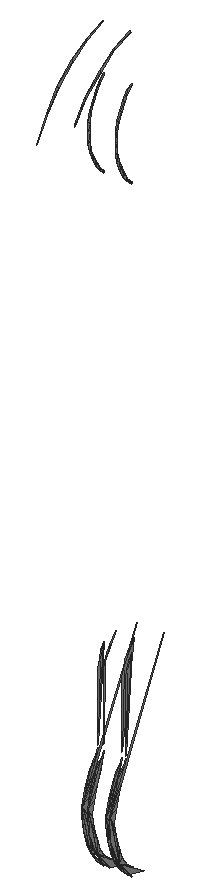
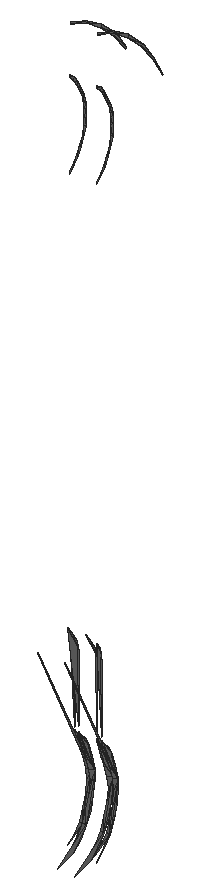
# SketchUp Ruby script. Lengths in inches.
U = 1.inch
M = Sketchup.active_model
def pt(a) = Geom::Point3d.new(a.map { |v| v * U })
def face(e, loops, mat)
  f = e.add_face(loops[0].map { |a| pt(a) })
  loops[1..].each { |l| e.add_face(l.map { |a| pt(a) }).erase! }
  f.material = f.back_material = mat if mat
  f
end
# faces: each face lists its corners as indices into pts; further lists are holes
def faces(e, pts, list, mat = nil) = list.each { |f| face(e, (f[0].is_a?(Array) ? f : [f]).map { |l| l.map { |i| pts[i] } }, mat) }
# xy, xz, yz: faces in a plane at the given z, y or x. An outline is a flat list of corners, or four numbers for a rectangle; further outlines are holes
def ring(l) = l.size == 4 ? [[l[0], l[1]], [l[2], l[1]], [l[2], l[3]], [l[0], l[3]]] : l.each_slice(2).to_a
def flat(e, list, mat, &to3) = list.each { |f| face(e, (f[0].is_a?(Array) ? f : [f]).map { |l| ring(l).map { |u, v| to3.(u, v) } }, mat) }
def xy(e, z, list, mat = nil) = flat(e, list, mat) { |x, y| [x, y, z] }
def xz(e, y, list, mat = nil) = flat(e, list, mat) { |x, z| [x, y, z] }
def yz(e, x, list, mat = nil) = flat(e, list, mat) { |y, z| [x, y, z] }
def lines(e, pts, list) = list.each { |a, b| e.add_line(pt(pts[a]), pt(pts[b])) }
# prism: a flat outline (further loops are holes) pulled along v
def prism(e, loops, v, mat = nil)
  f = face(e, loops, mat); d = Geom::Vector3d.new(v.map { |x| x * U })
  f.pushpull(f.normal.samedirection?(d) ? d.length : -d.length)
end
def box(e, o, s, mat = nil) = prism(e, [[o, [o[0] + s[0], o[1], o[2]], [o[0] + s[0], o[1] + s[1], o[2]], [o[0], o[1] + s[1], o[2]]]], [0, 0, s[2]], mat)
def at(x, y, z, deg = 0) = Geom::Transformation.translation(pt([x, y, z])) * Geom::Transformation.rotation(ORIGIN, Z_AXIS, deg.degrees)
def axes(o, x, y, z) = Geom::Transformation.new([*x, 0, *y, 0, *z, 0, *pt(o).to_a, 1])
def part(name) = M.definitions.add(name)
# library, detail: a bought-in or finely detailed component or shape, given as its bounding box
def library(name, o, s) = part(name).tap { |d| box(d.entities, o, s) }
def detail(e, o, s) = box(e.add_group.entities, o, s)
def put(e, d, t, mat = nil) = e.add_instance(d, t).tap { |i| i.material = mat if mat }
def group(e, t, mat = nil) = e.add_group.tap { |g| g.transformation = t; g.material = mat if mat }.entities
root = M.entities
M.materials.add("Material \#1").color = [140, 140, 140]
yz(root,263.95,[[328.065,58.084,328.018,58.124,327.978,58.176],[328.078,58.12,327.978,58.176,328.037,58.155],[328.037,58.155,327.978,58.176,328.002,58.201],[327.978,58.176,327.924,58.431,327.958,58.319],[327.978,58.176,327.929,58.31,327.924,58.431],
  [327.978,58.176,327.948,58.239,327.929,58.31],[327.978,58.176,327.958,58.319,327.975,58.256],[327.978,58.176,327.975,58.256,328.002,58.201],[327.929,58.31,327.922,58.387,327.924,58.431],[327.958,58.319,327.924,58.431,327.952,58.387],
  [327.952,58.387,327.924,58.431,327.958,58.455],[327.924,58.431,327.931,58.474,327.941,58.515],[327.924,58.431,327.941,58.515,327.973,58.588],[327.924,58.431,327.973,58.588,328.022,58.654],[327.924,58.431,327.975,58.517,327.958,58.455],
  [327.924,58.431,328.002,58.572,327.975,58.517],[327.924,58.431,328.022,58.654,328.026,58.66],[327.924,58.431,328.026,58.66,328.029,58.667],[327.924,58.431,328.288,59.173,328.002,58.572],[327.941,58.515,327.955,58.553,327.973,58.588],
  [327.973,58.588,327.994,58.62,328.017,58.648],[327.973,58.588,328.017,58.648,328.022,58.654],[328.034,58.6875,328.035,58.695,328.066,59.173],[328.035,58.695,328.035,59.055,328.038,59.098],[328.035,58.695,328.038,59.098,328.066,59.173],
  [328.038,59.098,328.049,59.138,328.066,59.173]],"Material \#1")
yz(root,263.952,[[328.067,61.457,328.037,61.485,328.044,61.497],[328.067,61.457,328.044,61.497,328.073,61.47],[328.037,61.485,328.011,61.52,328.019,61.53],[328.037,61.485,328.019,61.53,328.044,61.497],[328.011,61.52,327.989,61.56,327.999,61.568],
  [328.011,61.52,327.999,61.568,328.019,61.53],[327.989,61.56,327.973,61.605,327.984,61.61],[327.989,61.56,327.984,61.61,327.999,61.568],[327.973,61.605,327.963,61.654,327.974,61.657],[327.973,61.605,327.974,61.657,327.984,61.61],
  [327.963,61.654,327.959,61.71,327.971,61.71],[327.963,61.654,327.971,61.71,327.974,61.657],[327.959,61.71,327.963,61.757,327.974,61.754],[327.959,61.71,327.974,61.754,327.971,61.71],[327.974,61.754,327.963,61.757,327.984,61.8],
  [327.963,61.757,327.973,61.806,327.984,61.8],[327.984,61.8,327.973,61.806,327.999,61.843],[327.614,61.803,327.676,61.917,327.684,61.907],[327.973,61.806,327.989,61.851,327.999,61.843],[327.999,61.843,327.989,61.851,328.019,61.881],
  [327.989,61.851,328.011,61.891,328.019,61.881],[328.019,61.881,328.011,61.891,328.044,61.914],[328.011,61.891,328.037,61.925,328.044,61.914],[327.684,61.907,327.676,61.917,327.762,62.01],[328.044,61.914,328.037,61.925,328.073,61.941],
  [327.676,61.917,327.755,62.021,327.762,62.01],[328.037,61.925,328.067,61.954,328.073,61.941],[327.762,62.01,327.755,62.021,327.852,62.094],[327.755,62.021,327.846,62.107,327.852,62.094],[327.852,62.094,327.846,62.107,327.952,62.157],
  [327.846,62.107,327.948,62.171,327.952,62.157],[327.952,62.157,327.948,62.171,328.061,62.196],[327.948,62.171,328.059,62.211,328.061,62.196]],"Material \#1")
yz(root,263.975,[[328.177,58.05,327.978,58.176,328.065,58.084],[328.065,58.084,327.978,58.176,328.018,58.124],[328.078,58.12,328.037,58.155,327.978,58.176],[328.037,58.155,328.002,58.201,327.978,58.176],[327.978,58.176,327.924,58.431,327.929,58.31],
  [327.978,58.176,327.975,58.256,327.924,58.431],[327.978,58.176,327.929,58.31,327.948,58.239],[327.978,58.176,328.002,58.201,327.975,58.256],[327.975,58.256,327.958,58.319,327.924,58.431],[327.929,58.31,327.924,58.431,327.922,58.387],
  [327.958,58.319,327.952,58.387,327.924,58.431],[327.952,58.387,327.958,58.455,327.924,58.431],[327.924,58.431,327.941,58.515,327.931,58.474],[327.924,58.431,327.958,58.455,327.975,58.517],[327.924,58.431,327.973,58.588,327.941,58.515],
  [327.924,58.431,327.975,58.517,328.029,58.667],[327.924,58.431,328.022,58.654,327.973,58.588],[327.924,58.431,328.026,58.66,328.022,58.654],[327.924,58.431,328.029,58.667,328.026,58.66],[327.941,58.515,327.973,58.588,327.955,58.553],
  [327.975,58.517,328.002,58.572,328.029,58.667],[327.973,58.588,328.017,58.648,327.994,58.62],[327.973,58.588,328.022,58.654,328.017,58.648],[328.035,58.695,328.038,59.098,328.035,59.055],[328.038,59.098,328.066,59.173,328.049,59.138],
  [328.038,59.098,328.115,59.224,328.066,59.173]],"Material \#1")
yz(root,264.078,[[328.177,58.05,328.065,58.084,327.978,58.176],[328.065,58.084,328.018,58.124,327.978,58.176],[328.078,58.12,327.978,58.176,328.037,58.155],[328.037,58.155,327.978,58.176,328.002,58.201],[327.978,58.176,327.924,58.431,327.975,58.256],
  [327.978,58.176,327.929,58.31,327.924,58.431],[327.978,58.176,327.948,58.239,327.929,58.31],[327.978,58.176,327.975,58.256,328.002,58.201],[327.975,58.256,327.924,58.431,327.958,58.319],[327.929,58.31,327.922,58.387,327.924,58.431],
  [327.958,58.319,327.924,58.431,327.952,58.387],[327.952,58.387,327.924,58.431,327.958,58.455],[327.924,58.431,327.931,58.474,327.941,58.515],[327.924,58.431,327.941,58.515,327.973,58.588],[327.924,58.431,327.973,58.588,328.022,58.654],
  [327.924,58.431,327.975,58.517,327.958,58.455],[327.924,58.431,328.022,58.654,328.026,58.66],[327.924,58.431,328.026,58.66,328.029,58.667],[327.924,58.431,328.029,58.667,327.975,58.517],[327.941,58.515,327.955,58.553,327.973,58.588],
  [327.975,58.517,328.029,58.667,328.002,58.572],[327.973,58.588,327.994,58.62,328.017,58.648],[327.973,58.588,328.017,58.648,328.022,58.654],[328.035,58.695,328.035,59.055,328.038,59.098],[328.035,58.695,328.038,59.098,328.115,59.224],
  [328.038,59.098,328.049,59.138,328.066,59.173],[328.038,59.098,328.066,59.173,328.115,59.224],[328.066,59.173,328.088,59.202,328.115,59.224]],"Material \#1")
yz(root,264.101,[[328.067,61.457,328.044,61.497,328.037,61.485],[328.067,61.457,328.073,61.47,328.044,61.497],[328.037,61.485,328.019,61.53,328.011,61.52],[328.037,61.485,328.044,61.497,328.019,61.53],[328.011,61.52,327.999,61.568,327.989,61.56],
  [328.011,61.52,328.019,61.53,327.999,61.568],[327.989,61.56,327.984,61.61,327.973,61.605],[327.989,61.56,327.999,61.568,327.984,61.61],[327.973,61.605,327.974,61.657,327.963,61.654],[327.973,61.605,327.984,61.61,327.974,61.657],
  [327.963,61.654,327.971,61.71,327.959,61.71],[327.963,61.654,327.974,61.657,327.971,61.71],[327.959,61.71,327.971,61.71,327.974,61.754],[327.959,61.71,327.974,61.754,327.963,61.757],[327.974,61.754,327.984,61.8,327.963,61.757],
  [327.963,61.757,327.984,61.8,327.973,61.806],[327.984,61.8,327.999,61.843,327.973,61.806],[327.973,61.806,327.999,61.843,327.989,61.851],[327.999,61.843,328.019,61.881,327.989,61.851],[327.989,61.851,328.019,61.881,328.011,61.891],
  [328.019,61.881,328.044,61.914,328.011,61.891],[328.011,61.891,328.044,61.914,328.037,61.925],[327.684,61.907,327.762,62.01,327.676,61.917],[328.044,61.914,328.073,61.941,328.037,61.925],[327.676,61.917,327.762,62.01,327.755,62.021],
  [328.037,61.925,328.073,61.941,328.067,61.954],[327.762,62.01,327.852,62.094,327.755,62.021],[327.755,62.021,327.852,62.094,327.846,62.107],[327.852,62.094,327.952,62.157,327.846,62.107],[327.846,62.107,327.952,62.157,327.948,62.171],
  [327.952,62.157,328.061,62.196,327.948,62.171],[327.948,62.171,328.061,62.196,328.059,62.211]],"Material \#1")
yz(root,264.103,[[328.065,58.084,327.978,58.176,328.018,58.124],[328.078,58.12,328.037,58.155,327.978,58.176],[328.037,58.155,328.002,58.201,327.978,58.176],[327.978,58.176,327.924,58.431,327.929,58.31],[327.978,58.176,327.958,58.319,327.924,58.431],
  [327.978,58.176,327.929,58.31,327.948,58.239],[327.978,58.176,327.975,58.256,327.958,58.319],[327.978,58.176,328.002,58.201,327.975,58.256],[327.929,58.31,327.924,58.431,327.922,58.387],[327.958,58.319,327.952,58.387,327.924,58.431],
  [327.952,58.387,327.958,58.455,327.924,58.431],[327.924,58.431,327.941,58.515,327.931,58.474],[327.924,58.431,327.958,58.455,327.975,58.517],[327.924,58.431,327.973,58.588,327.941,58.515],[327.924,58.431,327.975,58.517,328.002,58.572],
  [327.924,58.431,328.002,58.572,328.288,59.173],[327.924,58.431,328.022,58.654,327.973,58.588],[327.924,58.431,328.026,58.66,328.022,58.654],[327.924,58.431,328.029,58.667,328.026,58.66],[327.941,58.515,327.973,58.588,327.955,58.553],
  [327.973,58.588,328.017,58.648,327.994,58.62],[327.973,58.588,328.022,58.654,328.017,58.648],[328.034,58.6875,328.066,59.173,328.035,58.695],[328.035,58.695,328.038,59.098,328.035,59.055],[328.035,58.695,328.066,59.173,328.038,59.098],
  [328.038,59.098,328.066,59.173,328.049,59.138]],"Material \#1")
